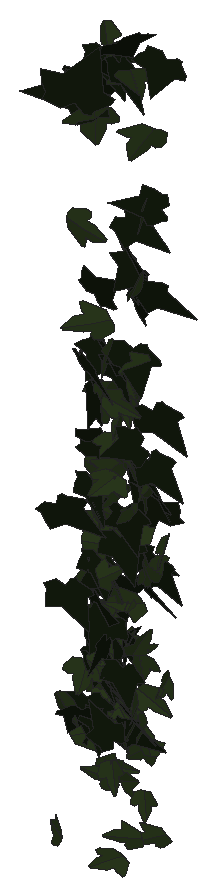
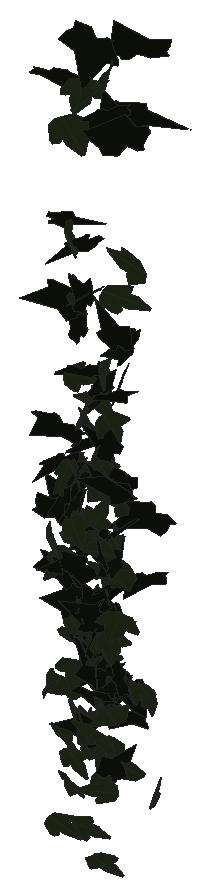
# SketchUp Ruby script. Lengths in inches.
U = 1.inch
M = Sketchup.active_model
def pt(a) = Geom::Point3d.new(a.map { |v| v * U })
def face(e, loops, mat)
  f = e.add_face(loops[0].map { |a| pt(a) })
  loops[1..].each { |l| e.add_face(l.map { |a| pt(a) }).erase! }
  f.material = f.back_material = mat if mat
  f
end
# faces: each face lists its corners as indices into pts; further lists are holes
def faces(e, pts, list, mat = nil) = list.each { |f| face(e, (f[0].is_a?(Array) ? f : [f]).map { |l| l.map { |i| pts[i] } }, mat) }
# xy, xz, yz: faces in a plane at the given z, y or x. An outline is a flat list of corners, or four numbers for a rectangle; further outlines are holes
def ring(l) = l.size == 4 ? [[l[0], l[1]], [l[2], l[1]], [l[2], l[3]], [l[0], l[3]]] : l.each_slice(2).to_a
def flat(e, list, mat, &to3) = list.each { |f| face(e, (f[0].is_a?(Array) ? f : [f]).map { |l| ring(l).map { |u, v| to3.(u, v) } }, mat) }
def xy(e, z, list, mat = nil) = flat(e, list, mat) { |x, y| [x, y, z] }
def xz(e, y, list, mat = nil) = flat(e, list, mat) { |x, z| [x, y, z] }
def yz(e, x, list, mat = nil) = flat(e, list, mat) { |y, z| [x, y, z] }
def lines(e, pts, list) = list.each { |a, b| e.add_line(pt(pts[a]), pt(pts[b])) }
# prism: a flat outline (further loops are holes) pulled along v
def prism(e, loops, v, mat = nil)
  f = face(e, loops, mat); d = Geom::Vector3d.new(v.map { |x| x * U })
  f.pushpull(f.normal.samedirection?(d) ? d.length : -d.length)
end
def box(e, o, s, mat = nil) = prism(e, [[o, [o[0] + s[0], o[1], o[2]], [o[0] + s[0], o[1] + s[1], o[2]], [o[0], o[1] + s[1], o[2]]]], [0, 0, s[2]], mat)
def at(x, y, z, deg = 0) = Geom::Transformation.translation(pt([x, y, z])) * Geom::Transformation.rotation(ORIGIN, Z_AXIS, deg.degrees)
def axes(o, x, y, z) = Geom::Transformation.new([*x, 0, *y, 0, *z, 0, *pt(o).to_a, 1])
def part(name) = M.definitions.add(name)
# library, detail: a bought-in or finely detailed component or shape, given as its bounding box
def library(name, o, s) = part(name).tap { |d| box(d.entities, o, s) }
def detail(e, o, s) = box(e.add_group.entities, o, s)
def put(e, d, t, mat = nil) = e.add_instance(d, t).tap { |i| i.material = mat if mat }
def group(e, t, mat = nil) = e.add_group.tap { |g| g.transformation = t; g.material = mat if mat }.entities
root = M.entities
M.materials.add("1026 AP 7946 SUNNY SIDE UP").color = [254, 231, 186]
M.materials.add("efeu1").color = [18, 25, 13]
M.materials.add("efeu2").color = [43, 57, 29]
c1 = part("ivyleaf_9")
p = [[1.54,2.16,1.25],[1.36,2.04,1.19],[-0.21,0.99,0.68],[-0.71,1.11,0.82],[-0.85,0.86,0.67],[-0.8,0.17,0.21],
  [-0.9,-0.01,0.1],[-0.67,-0.16,-0.02],[-0.08,-0.08,-0.05],[-0.03,-0.6,-0.4],[0.65,-0.88,-0.66],[0.83,-0.6,-0.49],
  [1.29,-0.42,-0.43],[1.8125,-0.07,-0.26],[1.21,0.44,0.15]]
faces(c1.entities,p,[[0,1,2,3,4,5,6,7,8,9,10,11,12,13,14]],"efeu1")
c2 = part("ivyleaf_10")
p = [[0,0.5,-0.03],[-0.0625,2.02,-0.43],[-0.19,2.01,-0.46],[-0.54,1.05,-0.29],[-0.52,0.625,-0.18],[-0.83,0.76,-0.28],
  [-1.16,0.64,-0.33],[-1.15,0.33,-0.24],[-0.77,-0.39,0.02],[-0.3,-0.51,0.16],[0.04,-0.48,0.23],[-0.02,2.01,-0.4375],
  [-0.06,2.01,-0.43],[0.04,-0.49,0.23],[0.67,-0.49,0.14],[1.38,0.36,-0.2],[1.375,0.51,-0.24],[0.81,0.65,-0.19],
  [0.62,0.59,-0.15],[0.6,1.09,-0.28],[0.5,1.23,-0.31]]
faces(c2.entities,p,[[0,1,2,3,4,5,6,7,8,9,10],[11,12,0,13,14,15,16,17,18,19,20]],"efeu2")
put(root,c1,axes([109.08,209.6,266.42],[-0.40684,-0.01544,0.2709],[0.40255,0.07255,0.26423],[-0.0981,0.36177,-0.03922]),"1026 AP 7946 SUNNY SIDE UP")
put(root,c2,axes([108.33,210.02,249.78],[-0.13693,0.19492,0.11799],[0.08574,-0.09978,0.21919],[0.34408,0.10243,-0.00767]),"1026 AP 7946 SUNNY SIDE UP")
put(root,c1,axes([109.52,210.18,252.23],[-0.23068,-0.18541,0.07834],[0.05778,0.06908,0.24358],[-0.31041,0.15065,-0.01287]),"1026 AP 7946 SUNNY SIDE UP")
put(root,c2,axes([109.09,210.38,261.2],[-0.16259,-0.02209,0.28134],[-0.26507,-0.22514,-0.08579],[0.33988,-0.18615,0.06768]),"1026 AP 7946 SUNNY SIDE UP")
put(root,c1,axes([108.63,210.39,260.22],[0.27928,-0.22573,0.03254],[0.01071,-0.03639,-0.29559],[0.35852,0.17693,-0.01652]),"1026 AP 7946 SUNNY SIDE UP")
put(root,c1,axes([108.28,210.34,255.07],[-0.02737,-0.23291,-0.15927],[0.047,0.15114,-0.2392],[0.4359,-0.03092,0.01579]),"1026 AP 7946 SUNNY SIDE UP")
put(root,c1,axes([108.74,210.59,259.36],[0.10963,-0.08572,-0.30104],[0.35309,-0.18728,0.11089],[-0.32236,-0.23429,0.01908]),"1026 AP 7946 SUNNY SIDE UP")
put(root,c1,axes([108.625,210.36,252.47],[0.11669,0.18455,-0.14395],[-0.06959,-0.13384,-0.20556],[-0.35828,0.0861,-0.00696]),"1026 AP 7946 SUNNY SIDE UP")
put(root,c2,axes([108.06,210.48,252.48],[-0.21918,0.105,-0.16969],[0.18108,-0.12018,-0.17937],[-0.24907,-0.17977,0.01892]),"1026 AP 7946 SUNNY SIDE UP")
put(root,c1,axes([109.03,210.57,254.01],[-0.0695,0.03995,-0.24484],[0.23279,-0.18646,-0.06168],[-0.29947,-0.15421,0.00888]),"1026 AP 7946 SUNNY SIDE UP")
put(root,c1,axes([109.43,210.62,253.54],[-0.05966,-0.24674,-0.05099],[0.01287,0.0474,-0.2569],[0.39507,-0.03881,0.00067]),"1026 AP 7946 SUNNY SIDE UP")
put(root,c1,axes([109.47,210.66,252.63],[0.2289,-0.16809,0.1221],[0.10463,-0.10013,-0.22925],[0.30692,0.1595,-0.01291]),"1026 AP 7946 SUNNY SIDE UP")
put(root,c1,axes([108.82,210.72,252.2],[-0.07424,-0.24072,0.04015],[-0.00793,-0.04012,-0.25294],[0.38371,-0.0474,0.00254]),"1026 AP 7946 SUNNY SIDE UP")
put(root,c1,axes([109.22,210.71,252.87],[0.27696,-0.1758,-0.02225],[0.04292,-0.00173,0.25569],[-0.27499,-0.17733,0.01751]),"1026 AP 7946 SUNNY SIDE UP")
put(root,c1,axes([107.96,210.5,256.7],[-0.00162,-0.0584,-0.28273],[0.19565,0.24553,-0.05293],[0.39488,-0.12189,0.02507]),"1026 AP 7946 SUNNY SIDE UP")
put(root,c2,axes([109.59,210.8,252.7],[-0.0379,0.06169,0.2687],[0.23938,-0.21195,0.06499],[0.3462,0.15331,-0.01552]),"1026 AP 7946 SUNNY SIDE UP")
put(root,c1,axes([108.5,210.8,265.8],[-0.1132,-0.14152,-0.30952],[-0.29108,-0.23715,0.15982],[-0.43218,0.19679,-0.02657]),"1026 AP 7946 SUNNY SIDE UP")
put(root,c2,axes([108.68,210.7,265.46],[-0.34074,-0.26216,-0.02461],[0.04806,0.00374,-0.34969],[0.41092,-0.21782,0.02049]),"1026 AP 7946 SUNNY SIDE UP")
put(root,c2,axes([109,210.79,251.15],[0.28995,-0.06537,0.14583],[0.19522,-0.072,-0.20077],[0.14918,0.22127,-0.02071]),"1026 AP 7946 SUNNY SIDE UP")
put(root,c2,axes([109.29,210.82,250.95],[-0.19761,0.04881,0.18853],[0.27608,-0.05143,0.13826],[0.11054,0.21572,-0.0083]),"1026 AP 7946 SUNNY SIDE UP")
put(root,c2,axes([108.93,210.9,250.83],[-0.00432,0.02959,0.24123],[-0.36452,-0.04343,0.0026],[0.0683,-0.22995,0.02913]),"1026 AP 7946 SUNNY SIDE UP")
put(root,c1,axes([108.73,211.09,254.2],[-0.25859,-0.20442,0.02913],[-0.00853,-0.03334,-0.26994],[0.32463,-0.16371,0.01611]),"1026 AP 7946 SUNNY SIDE UP")
put(root,c2,axes([108.16,211.01,252.98],[0.40102,-0.05002,0.02149],[0.02533,-0.02727,-0.2668],[0.08154,0.25446,-0.02281]),"1026 AP 7946 SUNNY SIDE UP")
put(root,c1,axes([108.26,211.03,252.29],[-0.18007,-0.1402,-0.1823],[0.22055,0.11017,-0.18362],[0.27692,-0.17891,0.0277]),"1026 AP 7946 SUNNY SIDE UP")
put(root,c2,axes([108.84,210.98,259.1],[0.05245,0.03506,0.24066],[0.36347,0.04278,-0.0404],[-0.07499,0.23187,-0.0275]),"1026 AP 7946 SUNNY SIDE UP")
put(root,c1,axes([108.4,211.15,254.23],[0.05286,-0.04592,0.26347],[0.15158,-0.23755,-0.05833],[0.37984,0.10119,-0.01339]),"1026 AP 7946 SUNNY SIDE UP")
put(root,c2,axes([108.78,210.83,255.27],[0.05699,0.00614,-0.24796],[0.16024,0.22018,0.02288],[0.34307,-0.10386,0.0305]),"1026 AP 7946 SUNNY SIDE UP")
put(root,c1,axes([109.19,210.8125,267.17],[0.19102,0.31859,0.04658],[0.04225,0.03618,-0.35083],[-0.50382,0.12383,-0.01176]),"1026 AP 7946 SUNNY SIDE UP")
put(root,c2,axes([109.68,211.125,265.21],[-0.26905,-0.23738,0.13623],[-0.09042,-0.12272,-0.30126],[0.41865,-0.17906,0.02248]),"1026 AP 7946 SUNNY SIDE UP")
put(root,c2,axes([109.24,210.92,251.79],[-0.07719,0.06912,0.2178],[-0.22129,0.15749,-0.08595],[-0.27009,-0.14879,0.00817]),"1026 AP 7946 SUNNY SIDE UP")
put(root,c2,axes([107.85,211.17,262.6],[-0.01694,-0.01772,-0.31642],[0.40086,-0.17238,0.00002],[-0.27053,-0.25432,0.01985]),"1026 AP 7946 SUNNY SIDE UP")
put(root,c1,axes([108.42,211.3,255.02],[0.09107,-0.14519,-0.21799],[0.13706,-0.192,0.1598],[-0.3784,-0.10449,0.00541]),"1026 AP 7946 SUNNY SIDE UP")
put(root,c1,axes([108.97,211.16,256.01],[-0.04179,-0.26634,-0.09699],[0.01818,0.09194,-0.27519],[0.44302,-0.0289,0.00214]),"1026 AP 7946 SUNNY SIDE UP")
put(root,c1,axes([109.27,211.29,258.11],[-0.21064,-0.10734,0.19768],[-0.18896,-0.15326,-0.17509],[0.29051,-0.17751,0.02945]),"1026 AP 7946 SUNNY SIDE UP")
put(root,c2,axes([109.41,211.1,253.74],[-0.11344,-0.23679,0.05939],[0.02996,0.05586,0.25533],[-0.38254,0.0746,0.00239]),"1026 AP 7946 SUNNY SIDE UP")
put(root,c2,axes([108.71,211.2,257.23],[0.25782,0.08648,-0.16174],[-0.19791,-0.09687,-0.19036],[-0.20161,0.20568,-0.01997]),"1026 AP 7946 SUNNY SIDE UP")
put(root,c2,axes([108.57,211.32,260.02],[0.10016,-0.19958,0.18834],[0.13189,-0.16523,-0.21556],[0.4059,0.10294,0.02356]),"1026 AP 7946 SUNNY SIDE UP")
put(root,c1,axes([108.34,211.28,255.29],[-0.03984,-0.26003,-0.02741],[0.006,0.02487,-0.269],[0.41073,-0.02559,0.00127]),"1026 AP 7946 SUNNY SIDE UP")
put(root,c2,axes([108.7,211.28,257.48],[-0.17686,-0.17198,0.1538],[-0.1099,-0.13355,-0.21213],[0.34188,-0.1319,0.01137]),"1026 AP 7946 SUNNY SIDE UP")
put(root,c2,axes([109.21,211.25,249.48],[-0.07293,-0.0047,0.21782],[-0.28336,-0.11247,-0.04395],[0.17413,-0.18499,0.01971]),"1026 AP 7946 SUNNY SIDE UP")
put(root,c1,axes([108.17,211.3,252.98],[0.16952,-0.24496,0.046],[0.01968,-0.04479,-0.2759],[0.39143,0.10834,-0.00605]),"1026 AP 7946 SUNNY SIDE UP")
put(root,c2,axes([108.76,211.25,248.87],[0.22778,0.0202,-0.1684],[-0.2504,-0.03898,-0.15047],[-0.0668,0.21499,-0.01015]),"1026 AP 7946 SUNNY SIDE UP")
put(root,c2,axes([108.24,211.33,256.15],[-0.18148,0.09939,0.22894],[0.24936,-0.15508,0.15579],[0.28936,0.19597,0.00933]),"1026 AP 7946 SUNNY SIDE UP")
put(root,c2,axes([109.21,211.2,266.31],[-0.28935,-0.21915,-0.06096],[0.09319,0.0255,-0.2932],[0.34403,-0.19123,0.02815]),"1026 AP 7946 SUNNY SIDE UP")
put(root,c2,axes([108.3,211.17,253.05],[-0.07178,-0.0703,-0.24089],[0.3671,0.05577,-0.06401],[0.11037,-0.23122,0.05625]),"1026 AP 7946 SUNNY SIDE UP")
put(root,c2,axes([109.17,211.27,251.99],[0.14149,-0.23736,-0.01979],[-0.02056,0.01413,-0.26132],[0.37372,0.09065,-0.00688]),"1026 AP 7946 SUNNY SIDE UP")
put(root,c1,axes([108.52,211.45,259.72],[-0.03945,-0.13299,0.2442],[0.07001,-0.2376,-0.13344],[0.42266,0.02694,0.0449]),"1026 AP 7946 SUNNY SIDE UP")
put(root,c2,axes([109.21,211.27,261.48],[0.00729,-0.24021,-0.00427],[0.00159,-0.00276,0.24749],[-0.37773,-0.00465,0.00096]),"1026 AP 7946 SUNNY SIDE UP")
put(root,c2,axes([109.45,211.21,252.07],[0.12757,-0.20528,-0.1121],[-0.07187,0.09765,-0.22674],[0.35732,0.09293,-0.00558]),"1026 AP 7946 SUNNY SIDE UP")
put(root,c1,axes([108.82,211.33,266.32],[0.15695,-0.27667,-0.04374],[-0.02602,0.0375,-0.30277],[0.43899,0.10114,-0.00231]),"1026 AP 7946 SUNNY SIDE UP")
put(root,c2,axes([109.39,211.32,250.41],[0.29095,-0.06022,0.1001],[0.13381,-0.05183,-0.19965],[0.1207,0.20263,-0.01995]),"1026 AP 7946 SUNNY SIDE UP")
put(root,c2,axes([109.25,211.17,257.67],[-0.01083,0.02822,0.25191],[-0.35552,0.09558,-0.01738],[-0.15237,-0.225,0.02264]),"1026 AP 7946 SUNNY SIDE UP")
put(root,c2,axes([108.43,211.35,251.57],[0.00284,-0.0206,-0.2238],[0.28904,-0.1167,0.0123],[-0.18455,-0.1831,0.01582]),"1026 AP 7946 SUNNY SIDE UP")
put(root,c1,axes([108.08,211.48,252.88],[0.00166,-0.18245,0.18515],[-0.0046,-0.18076,-0.18899],[0.40381,-0.00131,-0.00291]),"1026 AP 7946 SUNNY SIDE UP")
put(root,c1,axes([108.91,211.35,256.51],[-0.22536,-0.10421,-0.207],[0.29628,0.07561,-0.17894],[0.19573,-0.23444,0.03253]),"1026 AP 7946 SUNNY SIDE UP")
put(root,c2,axes([108.66,211.4375,250.72],[0.0121,-0.01301,-0.22023],[-0.1641,-0.18694,0.00676],[-0.29395,0.10383,-0.01284]),"1026 AP 7946 SUNNY SIDE UP")
put(root,c2,axes([109.47,211.37,255.32],[-0.16072,0.18468,0.13104],[0.10887,-0.10575,0.21667],[0.33439,0.1232,-0.00757]),"1026 AP 7946 SUNNY SIDE UP")
put(root,c1,axes([108.25,211.41,252.91],[0.18833,-0.16625,0.14467],[0.11432,-0.12165,-0.21155],[0.32354,0.13976,-0.00946]),"1026 AP 7946 SUNNY SIDE UP")
put(root,c1,axes([108.86,211.27,251.79],[0.09856,-0.01313,-0.24365],[0.29774,0.14965,0.04403],[0.22359,-0.19349,0.04877]),"1026 AP 7946 SUNNY SIDE UP")
put(root,c2,axes([109.46,211.5,257.3],[-0.0018,-0.06477,0.26051],[0.12789,-0.24076,-0.06447],[0.39061,0.07853,0.02231]),"1026 AP 7946 SUNNY SIDE UP")
put(root,c2,axes([108.62,211.375,257.96],[0.28834,0.11363,-0.09089],[-0.10254,-0.06291,-0.22186],[-0.20232,0.19382,-0.01709]),"1026 AP 7946 SUNNY SIDE UP")
put(root,c2,axes([108.8125,211.24,254.67],[-0.24788,0.15841,-0.13894],[-0.12605,0.11111,0.2301],[0.30286,0.1759,-0.01795]),"1026 AP 7946 SUNNY SIDE UP")
put(root,c2,axes([108.05,211.4,257.27],[-0.02752,-0.00856,-0.2364],[0.30125,-0.12732,-0.01091],[-0.19891,-0.19165,0.01618]),"1026 AP 7946 SUNNY SIDE UP")
put(root,c2,axes([108.36,211.35,254.22],[-0.21036,0.02482,-0.1825],[0.25789,-0.07172,-0.13826],[-0.11282,-0.21021,0.02423]),"1026 AP 7946 SUNNY SIDE UP")
put(root,c2,axes([109.23,211.5,259.83],[-0.02591,-0.08032,0.22901],[-0.08455,-0.21619,-0.08567],[0.3626,-0.05615,-0.00361]),"1026 AP 7946 SUNNY SIDE UP")
put(root,c2,axes([108.15,211.45,256.28],[0.07256,-0.0813,-0.22049],[0.21158,-0.16643,0.09425],[-0.29042,-0.14156,0.01358]),"1026 AP 7946 SUNNY SIDE UP")
put(root,c2,axes([108.64,211.48,256.71],[-0.12355,-0.14894,-0.16831],[-0.09061,-0.15267,0.17194],[-0.3346,0.09634,0.01559]),"1026 AP 7946 SUNNY SIDE UP")
put(root,c2,axes([108.38,211.43,259.05],[-0.1265,-0.24412,0.08692],[-0.01747,-0.08647,-0.26481],[0.40648,-0.07969,0.01567]),"1026 AP 7946 SUNNY SIDE UP")
put(root,c2,axes([108.4375,211.375,266.96],[-0.02232,0.27481,-0.08241],[0.00505,-0.08149,-0.28396],[-0.45071,-0.01452,0.0009]),"1026 AP 7946 SUNNY SIDE UP")
put(root,c2,axes([109.27,211.48,256.91],[-0.18704,0.09503,0.21731],[0.20969,-0.16492,0.15344],[0.29633,0.17669,0.02859]),"1026 AP 7946 SUNNY SIDE UP")
put(root,c2,axes([108.1,211.34,255.57],[0.0802,-0.05716,-0.25557],[0.39826,-0.01071,0.0562],[-0.03502,-0.25272,0.05387]),"1026 AP 7946 SUNNY SIDE UP")
put(root,c2,axes([109.12,211.37,254.58],[0.1705,-0.02426,-0.22526],[-0.34279,0.01974,-0.11358],[0.04484,0.24314,-0.0118]),"1026 AP 7946 SUNNY SIDE UP")
put(root,c2,axes([108.99,211.43,253.77],[0.17805,-0.21473,0.03841],[0.01617,-0.03808,-0.25015],[0.34264,0.11338,-0.00816]),"1026 AP 7946 SUNNY SIDE UP")
put(root,c1,axes([109.01,211.46,260.04],[-0.15365,-0.25082,-0.10774],[0.08053,0.09061,-0.27641],[0.41877,-0.10945,0.01362]),"1026 AP 7946 SUNNY SIDE UP")
put(root,c1,axes([108.98,211.58,257.375],[0.22798,-0.15625,-0.18343],[0.2199,-0.11076,0.21788],[-0.29935,-0.20036,0.02036]),"1026 AP 7946 SUNNY SIDE UP")
put(root,c2,axes([108.79,211.47,258.87],[0.25992,-0.05506,0.15958],[0.21189,-0.08121,-0.178],[0.14887,0.21171,-0.02527]),"1026 AP 7946 SUNNY SIDE UP")
put(root,c1,axes([108.68,211.58,253.5],[-0.06328,-0.15583,0.18696],[-0.02876,-0.18238,-0.16577],[0.37608,-0.04017,0.01878]),"1026 AP 7946 SUNNY SIDE UP")
put(root,c1,axes([107.99,211.5,256.77],[0.03084,-0.27394,-0.00899],[-0.0043,0.00699,-0.28288],[0.43087,0.01968,-0.00218]),"1026 AP 7946 SUNNY SIDE UP")
put(root,c2,axes([107.77,211.35,251.22],[0.21122,-0.03362,-0.20063],[0.31024,0.01395,0.13793],[-0.01174,-0.23601,0.03532]),"1026 AP 7946 SUNNY SIDE UP")
put(root,c2,axes([109.13,211.37,256],[0.30511,0.14346,0.10915],[-0.17174,-0.0267,0.24503],[0.22073,-0.21907,0.03977]),"1026 AP 7946 SUNNY SIDE UP")
put(root,c2,axes([108.49,211.46,253.59],[0.25294,0.17907,-0.12333],[-0.11113,-0.0986,-0.24825],[-0.32088,0.1753,-0.01124]),"1026 AP 7946 SUNNY SIDE UP")
put(root,c1,axes([108.25,211.56,259.76],[-0.22642,-0.1921,0.04872],[-0.02034,-0.05058,-0.24679],[0.31083,-0.14324,0.01935]),"1026 AP 7946 SUNNY SIDE UP")
put(root,c2,axes([108.4375,211.35,253.52],[0.17547,-0.02917,-0.21802],[0.33454,0.03464,0.11095],[0.02734,-0.23658,0.04169]),"1026 AP 7946 SUNNY SIDE UP")
put(root,c1,axes([108.09,211.48,260.99],[-0.12572,0.03278,0.26663],[0.2332,-0.21676,0.07427],[0.33713,0.16216,0.04806]),"1026 AP 7946 SUNNY SIDE UP")
put(root,c2,axes([109.11,211.34,256.62],[-0.13852,-0.19897,-0.12648],[0.10346,0.10354,-0.22296],[0.3518,-0.1088,0.01577]),"1026 AP 7946 SUNNY SIDE UP")
put(root,c1,axes([108.47,211.5,259.55],[0.13266,-0.23848,0.01195],[-0.00097,-0.01395,-0.26063],[0.37553,0.08421,-0.0049]),"1026 AP 7946 SUNNY SIDE UP")
put(root,c1,axes([108.64,211.5,254.76],[-0.02687,-0.04507,0.24775],[0.26416,-0.17777,-0.02304],[0.28026,0.16324,0.04547]),"1026 AP 7946 SUNNY SIDE UP")
put(root,c1,axes([109.52,211.38,257.81],[0.07893,-0.21043,-0.19424],[0.00105,0.19039,-0.21901],[0.44303,0.03704,0.03512]),"1026 AP 7946 SUNNY SIDE UP")
put(root,c1,axes([109.11,211.45,257.67],[0.2291,-0.19977,-0.04196],[-0.04513,0.02806,-0.25447],[0.31703,0.14835,-0.0059]),"1026 AP 7946 SUNNY SIDE UP")
put(root,c2,axes([108.48,211.3,252.2],[0.16887,0.17513,-0.12802],[0.07121,0.11847,0.21134],[0.33099,-0.11484,0.01985]),"1026 AP 7946 SUNNY SIDE UP")
put(root,c1,axes([108.53,211.47,253.75],[0.20221,-0.01739,-0.22288],[0.3377,0.04573,0.12806],[0.04821,-0.2474,0.03783]),"1026 AP 7946 SUNNY SIDE UP")
put(root,c2,axes([109.35,211.38,252.625],[0.17801,0.06784,0.2058],[0.29315,0.07303,-0.13422],[-0.15407,0.21734,-0.0176]),"1026 AP 7946 SUNNY SIDE UP")
put(root,c1,axes([108.92,211.66,261.75],[-0.17291,-0.17805,0.16935],[-0.06344,-0.16565,-0.21231],[0.37683,-0.10959,0.04197]),"1026 AP 7946 SUNNY SIDE UP")
put(root,c1,axes([109.72,211.57,266.63],[-0.30114,-0.17236,-0.04263],[0.07452,0.00743,-0.26405],[0.2682,-0.19559,0.0255]),"1026 AP 7946 SUNNY SIDE UP")
put(root,c1,axes([107.93,211.48,265.58],[0.49574,0.09113,0.06527],[-0.1116,0.02084,0.33581],[0.13358,-0.3208,0.03832]),"1026 AP 7946 SUNNY SIDE UP")
put(root,c2,axes([109.59,211.32,255.54],[-0.12795,-0.19554,-0.20155],[0.15283,0.16949,-0.2164],[0.40589,-0.12545,0.01794]),"1026 AP 7946 SUNNY SIDE UP")
put(root,c1,axes([107.91,211.54,253.42],[0.07394,-0.04982,-0.24668],[0.38258,-0.01238,0.05187],[-0.03459,-0.24343,0.04636]),"1026 AP 7946 SUNNY SIDE UP")
put(root,c2,axes([109.62,211.52,249.55],[-0.1637,-0.06439,0.18901],[-0.22221,-0.11848,-0.12589],[0.21078,-0.17491,0.01407]),"1026 AP 7946 SUNNY SIDE UP")
put(root,c2,axes([108.27,211.42,252.34],[-0.23804,-0.16985,0.10597],[0.08834,0.08868,0.23437],[-0.3003,0.16073,-0.01505]),"1026 AP 7946 SUNNY SIDE UP")
put(root,c1,axes([108.85,211.35,253.66],[0.09389,-0.03553,-0.24679],[-0.35745,0.07625,-0.06964],[0.13039,0.23461,-0.01319]),"1026 AP 7946 SUNNY SIDE UP")
put(root,c1,axes([108.19,211.4,257.48],[-0.18061,0.08217,0.21535],[0.308,-0.07718,0.142],[0.17142,0.22525,-0.02825]),"1026 AP 7946 SUNNY SIDE UP")
put(root,c2,axes([108.3,211.375,251.71],[-0.16229,-0.11462,-0.15901],[0.19234,0.09505,-0.15709],[0.23215,-0.15887,0.01899]),"1026 AP 7946 SUNNY SIDE UP")
put(root,c1,axes([109.55,211.57,263.32],[-0.23991,-0.00006,0.19365],[-0.28527,-0.0633,-0.1521],[0.07734,-0.23368,0.03968]),"1026 AP 7946 SUNNY SIDE UP")
put(root,c2,axes([108.29,211.5,256.12],[0.19031,0.019,0.25552],[0.39098,-0.00855,-0.12442],[-0.00098,0.27576,-0.01984]),"1026 AP 7946 SUNNY SIDE UP")
put(root,c1,axes([108.58,211.66,254.08],[0.00317,-0.04885,-0.25006],[0.24958,-0.18569,0.03882],[-0.29824,-0.15591,0.02982]),"1026 AP 7946 SUNNY SIDE UP")
put(root,c2,axes([109.67,211.62,256],[0.19687,-0.14205,0.18278],[0.14763,-0.15315,-0.19458],[0.32655,0.15488,-0.02222]),"1026 AP 7946 SUNNY SIDE UP")
put(root,c1,axes([108.93,211.64,260.98],[0.03054,-0.06039,0.25989],[0.08988,-0.24612,-0.06658],[0.3984,0.06015,-0.0049]),"1026 AP 7946 SUNNY SIDE UP")
put(root,c2,axes([108.5,211.65,258.32],[-0.0252,-0.10502,0.22097],[0.1717,-0.19504,-0.09086],[0.33491,0.09209,0.06321]),"1026 AP 7946 SUNNY SIDE UP")
put(root,c1,axes([109.59,211.52,256.53],[0.19671,0.02752,0.24913],[-0.379,0.05053,0.12291],[-0.05137,-0.2674,0.04723]),"1026 AP 7946 SUNNY SIDE UP")
put(root,c1,axes([109.34,211.43,261.52],[0.0714,-0.00115,-0.27704],[0.30981,0.18576,0.03454],[0.28779,-0.19968,0.03154]),"1026 AP 7946 SUNNY SIDE UP")
put(root,c1,axes([108.95,211.38,262.96],[0.16288,-0.15137,-0.23971],[-0.02471,0.2439,-0.16988],[0.43464,0.07059,0.08017]),"1026 AP 7946 SUNNY SIDE UP")
put(root,c1,axes([108.14,211.61,251.2],[0.07492,0.05535,0.24204],[-0.30669,-0.13171,0.07204],[0.22278,-0.19994,0.01778]),"1026 AP 7946 SUNNY SIDE UP")
put(root,c2,axes([109.47,211.43,251.44],[0.27706,-0.04396,0.12406],[-0.1734,0.05323,0.18617],[-0.10352,-0.20682,0.0202]),"1026 AP 7946 SUNNY SIDE UP")
put(root,c1,axes([109.34,211.65,256.95],[0.264,-0.08787,-0.2256],[0.33423,-0.05895,0.19235],[-0.15938,-0.26916,0.0297]),"1026 AP 7946 SUNNY SIDE UP")
put(root,c2,axes([108.52,211.53,253.96],[0.02395,-0.25178,-0.01353],[0.0164,-0.01109,0.2596],[-0.39598,-0.01569,0.00993]),"1026 AP 7946 SUNNY SIDE UP")
put(root,c2,axes([108.26,211.5,254.17],[-0.18063,-0.21376,-0.0055],[0.01797,-0.00146,-0.24976],[0.3357,-0.11494,0.01041]),"1026 AP 7946 SUNNY SIDE UP")
put(root,c2,axes([108.91,211.46,254.44],[0.20633,-0.20123,0.05395],[-0.02886,0.05183,0.24745],[-0.32614,-0.1319,0.01224]),"1026 AP 7946 SUNNY SIDE UP")
put(root,c1,axes([108.39,211.63,256.15],[-0.10249,-0.01058,-0.27801],[0.41258,-0.06797,-0.06296],[-0.10018,-0.26911,0.02516]),"1026 AP 7946 SUNNY SIDE UP")
put(root,c1,axes([108.65,211.61,252.86],[-0.31271,-0.12408,-0.09048],[0.13247,0.02903,-0.24055],[0.19821,-0.21517,0.01802]),"1026 AP 7946 SUNNY SIDE UP")
put(root,c1,axes([108.42,211.48,253.3],[0.28072,0.19986,0.02649],[-0.05279,-0.00284,0.27503],[0.31219,-0.18019,0.02269]),"1026 AP 7946 SUNNY SIDE UP")
put(root,c1,axes([109.47,211.58,255.4],[-0.04977,-0.0654,-0.25713],[0.3941,0.05043,-0.04613],[0.09397,-0.24611,0.05728]),"1026 AP 7946 SUNNY SIDE UP")
put(root,c2,axes([109.26,211.375,257.625],[0.01693,-0.07166,-0.23499],[-0.14122,0.20997,-0.07122],[0.34777,0.08875,-0.01748]),"1026 AP 7946 SUNNY SIDE UP")
put(root,c1,axes([107.9,211.45,257.67],[0.19391,0.023,0.22032],[0.338,-0.01481,-0.12622],[0.00221,0.24631,-0.02671]),"1026 AP 7946 SUNNY SIDE UP")
put(root,c2,axes([107.87,211.56,255.9],[-0.25879,0.02421,-0.21805],[0.31385,-0.07646,-0.16924],[-0.11771,-0.2571,0.02815]),"1026 AP 7946 SUNNY SIDE UP")
put(root,c2,axes([109.38,211.4375,257.64],[-0.07791,-0.20713,-0.17543],[0.10676,0.15661,-0.21718],[0.40667,-0.0808,0.0234]),"1026 AP 7946 SUNNY SIDE UP")
put(root,c2,axes([108.61,211.5625,251.92],[0.31197,0.05629,0.14365],[0.22171,0.00905,-0.21088],[-0.0808,0.24215,-0.02401]),"1026 AP 7946 SUNNY SIDE UP")
put(root,c1,axes([108.98,211.45,255.58],[0.07501,-0.01552,-0.25126],[0.18377,0.21959,0.01044],[0.33733,-0.11618,0.05018]),"1026 AP 7946 SUNNY SIDE UP")
put(root,c2,axes([108.01,211.55,254.72],[-0.32256,-0.11697,-0.07156],[0.1123,0.01298,-0.24203],[0.18145,-0.21598,0.02257]),"1026 AP 7946 SUNNY SIDE UP")
put(root,c2,axes([109.125,211.57,253.28],[-0.36742,0.01515,0.0115],[-0.01979,-0.02384,-0.24003],[-0.02189,-0.23271,0.02396]),"1026 AP 7946 SUNNY SIDE UP")
put(root,c2,axes([108.32,211.46,250.64],[0.00756,-0.00576,0.24074],[0.23252,0.18113,0.00252],[-0.28473,0.14777,0.00845]),"1026 AP 7946 SUNNY SIDE UP")
put(root,c2,axes([109.08,211.65,256.58],[-0.10875,-0.2371,0.05535],[-0.00565,-0.05626,-0.25447],[0.38271,-0.0682,0.01197]),"1026 AP 7946 SUNNY SIDE UP")
put(root,c1,axes([108.2,211.65,266.27],[-0.01993,-0.27065,-0.13957],[0.01308,0.13369,-0.27834],[0.47465,-0.01505,0.00181]),"1026 AP 7946 SUNNY SIDE UP")
put(root,c2,axes([109.19,211.59,251.26],[-0.25722,0.02718,0.16013],[-0.2474,-0.01412,-0.16828],[-0.01553,-0.22511,0.02855]),"1026 AP 7946 SUNNY SIDE UP")
put(root,c2,axes([108.94,211.58,258.9375],[-0.10429,0.23342,-0.01422],[-0.01054,0.01383,0.25006],[0.36766,0.06661,0.00313]),"1026 AP 7946 SUNNY SIDE UP")
put(root,c1,axes([108.67,211.78,261.81],[0.06937,-0.09032,0.24643],[0.11601,-0.22846,-0.104],[0.38574,0.08496,-0.01304]),"1026 AP 7946 SUNNY SIDE UP")
put(root,c1,axes([109.39,211.64,258.75],[-0.1085,-0.11762,-0.25571],[0.31342,0.15366,-0.13156],[0.29577,-0.20598,0.0456]),"1026 AP 7946 SUNNY SIDE UP")
put(root,c1,axes([108.05,211.72,258.61],[0.10726,-0.05555,0.23534],[0.21265,-0.1857,-0.08909],[0.30298,0.15,-0.02079]),"1026 AP 7946 SUNNY SIDE UP")
put(root,c1,axes([108.47,211.48,254.5],[-0.03122,0.00562,0.2908],[0.41827,0.09512,0.01788],[-0.14864,0.26648,-0.01076]),"1026 AP 7946 SUNNY SIDE UP")
put(root,c1,axes([109.03,211.69,254.84],[0.27229,-0.13973,0.11668],[0.11841,-0.08766,-0.22894],[0.25771,0.18791,-0.01809]),"1026 AP 7946 SUNNY SIDE UP")
put(root,c1,axes([108.06,211.76,255.91],[0.22993,-0.2042,-0.00348],[0.02347,0.00797,0.25821],[-0.32024,-0.14603,0.01643]),"1026 AP 7946 SUNNY SIDE UP")
put(root,c2,axes([109.08,211.78,263.2],[0.19103,-0.22206,0.15841],[0.12124,-0.13451,-0.26154],[0.40822,0.14387,0.00355]),"1026 AP 7946 SUNNY SIDE UP")
put(root,c2,axes([109.6,211.8,252.82],[0.02727,0.07558,-0.23013],[-0.04114,-0.22242,-0.08077],[-0.36916,0.03037,-0.008]),"1026 AP 7946 SUNNY SIDE UP")
put(root,c1,axes([108.91,211.85,257.06],[-0.00784,-0.11806,0.2367],[0.00558,-0.23049,-0.12292],[0.40708,0.00089,0.00624]),"1026 AP 7946 SUNNY SIDE UP")
put(root,c2,axes([108.32,211.5,258.45],[-0.01211,-0.01469,-0.2373],[-0.15586,0.20825,-0.00905],[0.32761,0.09854,-0.01308]),"1026 AP 7946 SUNNY SIDE UP")
